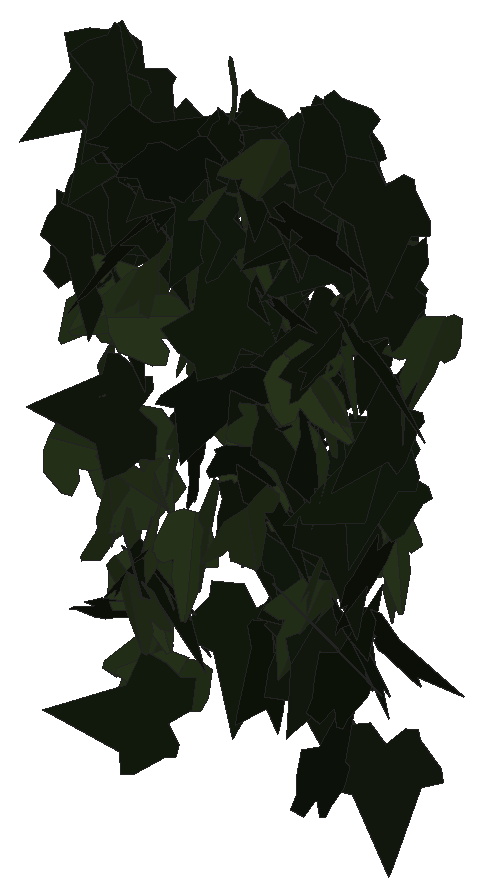
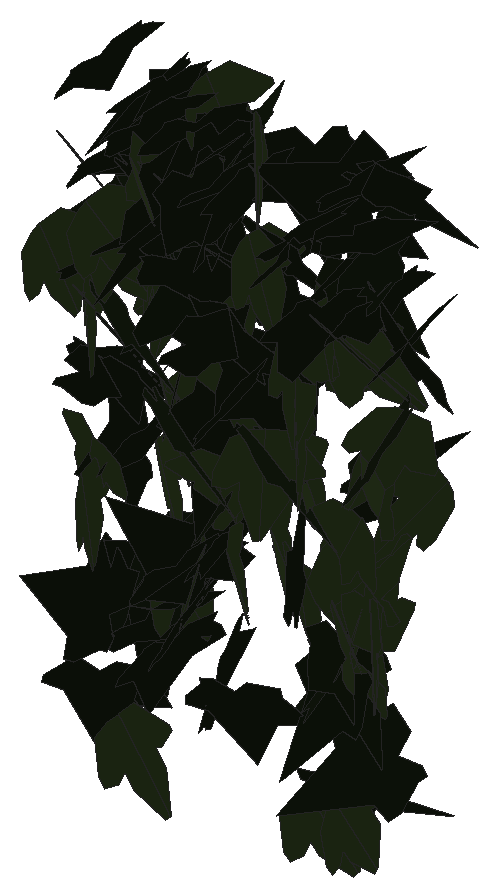
# SketchUp Ruby script. Lengths in inches.
U = 1.inch
M = Sketchup.active_model
def pt(a) = Geom::Point3d.new(a.map { |v| v * U })
def face(e, loops, mat)
  f = e.add_face(loops[0].map { |a| pt(a) })
  loops[1..].each { |l| e.add_face(l.map { |a| pt(a) }).erase! }
  f.material = f.back_material = mat if mat
  f
end
# faces: each face lists its corners as indices into pts; further lists are holes
def faces(e, pts, list, mat = nil) = list.each { |f| face(e, (f[0].is_a?(Array) ? f : [f]).map { |l| l.map { |i| pts[i] } }, mat) }
# xy, xz, yz: faces in a plane at the given z, y or x. An outline is a flat list of corners, or four numbers for a rectangle; further outlines are holes
def ring(l) = l.size == 4 ? [[l[0], l[1]], [l[2], l[1]], [l[2], l[3]], [l[0], l[3]]] : l.each_slice(2).to_a
def flat(e, list, mat, &to3) = list.each { |f| face(e, (f[0].is_a?(Array) ? f : [f]).map { |l| ring(l).map { |u, v| to3.(u, v) } }, mat) }
def xy(e, z, list, mat = nil) = flat(e, list, mat) { |x, y| [x, y, z] }
def xz(e, y, list, mat = nil) = flat(e, list, mat) { |x, z| [x, y, z] }
def yz(e, x, list, mat = nil) = flat(e, list, mat) { |y, z| [x, y, z] }
def lines(e, pts, list) = list.each { |a, b| e.add_line(pt(pts[a]), pt(pts[b])) }
# prism: a flat outline (further loops are holes) pulled along v
def prism(e, loops, v, mat = nil)
  f = face(e, loops, mat); d = Geom::Vector3d.new(v.map { |x| x * U })
  f.pushpull(f.normal.samedirection?(d) ? d.length : -d.length)
end
def box(e, o, s, mat = nil) = prism(e, [[o, [o[0] + s[0], o[1], o[2]], [o[0] + s[0], o[1] + s[1], o[2]], [o[0], o[1] + s[1], o[2]]]], [0, 0, s[2]], mat)
def at(x, y, z, deg = 0) = Geom::Transformation.translation(pt([x, y, z])) * Geom::Transformation.rotation(ORIGIN, Z_AXIS, deg.degrees)
def axes(o, x, y, z) = Geom::Transformation.new([*x, 0, *y, 0, *z, 0, *pt(o).to_a, 1])
def part(name) = M.definitions.add(name)
# library, detail: a bought-in or finely detailed component or shape, given as its bounding box
def library(name, o, s) = part(name).tap { |d| box(d.entities, o, s) }
def detail(e, o, s) = box(e.add_group.entities, o, s)
def put(e, d, t, mat = nil) = e.add_instance(d, t).tap { |i| i.material = mat if mat }
def group(e, t, mat = nil) = e.add_group.tap { |g| g.transformation = t; g.material = mat if mat }.entities
root = M.entities
M.materials.add("efeu1").color = [18, 25, 13]
M.materials.add("efeu2").color = [43, 57, 29]
c1 = part("ivyleaf_9")
p = [[1.54,2.16,1.25],[1.36,2.04,1.19],[-0.21,0.99,0.68],[-0.71,1.11,0.82],[-0.85,0.86,0.67],[-0.8,0.17,0.21],
  [-0.9,-0.01,0.1],[-0.67,-0.16,-0.02],[-0.08,-0.08,-0.05],[-0.03,-0.6,-0.4],[0.65,-0.88,-0.66],[0.83,-0.6,-0.49],
  [1.29,-0.42,-0.43],[1.8125,-0.07,-0.26],[1.21,0.44,0.15]]
faces(c1.entities,p,[[0,1,2,3,4,5,6,7,8,9,10,11,12,13,14]],"efeu1")
c2 = part("ivyleaf_10")
p = [[0,0.5,-0.03],[-0.0625,2.02,-0.43],[-0.19,2.01,-0.46],[-0.54,1.05,-0.29],[-0.52,0.625,-0.18],[-0.83,0.76,-0.28],
  [-1.16,0.64,-0.33],[-1.15,0.33,-0.24],[-0.77,-0.39,0.02],[-0.3,-0.51,0.16],[0.04,-0.48,0.23],[-0.02,2.01,-0.4375],
  [-0.06,2.01,-0.43],[0.04,-0.49,0.23],[0.67,-0.49,0.14],[1.38,0.36,-0.2],[1.375,0.51,-0.24],[0.81,0.65,-0.19],
  [0.62,0.59,-0.15],[0.6,1.09,-0.28],[0.5,1.23,-0.31]]
faces(c2.entities,p,[[0,1,2,3,4,5,6,7,8,9,10],[11,12,0,13,14,15,16,17,18,19,20]],"efeu2")
put(root,c1,axes([43.79,221.11,233.95],[-0.00332,-0.19199,0.46166],[0.22694,0.41079,0.17247],[-0.44552,0.21068,0.08441]))
put(root,c1,axes([40.89,221.49,240.28],[-0.2736,0.29374,-0.29809],[0.10434,-0.29702,-0.38845],[-0.40529,-0.27476,0.10123]))
put(root,c2,axes([42.59,221.28,237.12],[-0.08514,-0.46308,-0.16825],[0.01385,0.16843,-0.47057],[0.4925,-0.08479,-0.01586]))
put(root,c1,axes([44.14,221.52,239.85],[0.30164,-0.34888,0.19313],[0.13676,-0.13697,-0.46102],[0.37458,0.33095,0.0128]))
put(root,c2,axes([40.13,221.02,237.35],[0.08244,0.21818,0.44227],[-0.01318,0.44922,-0.21916],[-0.49298,0.02448,0.07982]))
put(root,c1,axes([40.54,221.77,237.6],[-0.02326,-0.39145,-0.31021],[0.04367,-0.31095,0.38911],[-0.49755,-0.00899,0.04865]))
put(root,c2,axes([43.27,221.34,239.25],[0.30785,0.09798,0.38161],[0.35199,0.14918,-0.32226],[-0.17701,0.46706,0.02288]))
put(root,c1,axes([43.21,221.79,237.81],[-0.00876,-0.11105,0.48743],[-0.01948,-0.48706,-0.11131],[0.49954,-0.02094,0.00421]))
put(root,c2,axes([40.78,221.57,239.25],[-0.24883,-0.09733,0.42262],[-0.34608,-0.24908,-0.26113],[0.26136,-0.42248,0.05659]))
put(root,c1,axes([43.24,221.3,241.21],[0.47749,-0.04289,0.14201],[0.14143,-0.01284,-0.47941],[0.04477,0.49799,-0.00013]))
put(root,c1,axes([43.92,221.33,239.99],[-0.31221,0.38447,0.06861],[-0.07065,0.03078,-0.49403],[-0.3841,-0.31817,0.0351]))
put(root,c2,axes([42.76,221.57,241.85],[-0.10777,-0.46898,0.13582],[-0.03653,-0.13095,-0.48116],[0.48688,-0.11364,-0.00603]))
put(root,c1,axes([43.64,221.35,239.74],[-0.36383,0.30082,0.16472],[-0.12248,0.11034,-0.47204],[-0.32035,-0.38384,-0.0066]))
put(root,c1,axes([44.3,221.7,241.87],[-0.02942,-0.498,0.03368],[-0.00026,-0.03372,-0.49886],[0.49913,-0.02937,0.00173]))
put(root,c1,axes([41.48,221.4,241.5],[0.13266,0.40843,-0.2561],[-0.06163,-0.24907,-0.42915],[-0.47812,0.14543,-0.01574]))
put(root,c1,axes([42.04,221.47,238.62],[0.07005,0.38741,-0.30823],[-0.05423,-0.30342,-0.39369],[-0.49209,0.08858,-0.00049]))
put(root,c2,axes([43.5,221.41,239.17],[-0.44305,0.23175,0.00106],[-0.00096,0.00047,-0.5],[-0.23175,-0.44305,0.00003]))
put(root,c1,axes([39.86,221.8,239.75],[0.04664,-0.47589,0.14612],[0.03164,-0.14363,-0.47788],[0.49681,0.05383,0.01672]))
put(root,c2,axes([41.12,221.46,239.87],[-0.00839,-0.48505,-0.12106],[0.01583,0.12076,-0.48494],[0.49968,-0.01197,0.01333]))
put(root,c1,axes([43.64,221.73,237.31],[0.07326,-0.49423,-0.01927],[-0.00281,0.01907,-0.49963],[0.4946,0.07331,0.00001]))
put(root,c2,axes([40.79,221.35,239.07],[-0.0798,-0.05196,0.49085],[0.3641,0.32952,0.09407],[-0.33326,0.37245,-0.01475]))
put(root,c1,axes([42.3,221.49,239.24],[-0.46284,-0.17411,0.07395],[0.07953,-0.00177,0.49363],[-0.17163,0.4687,0.02933]))
put(root,c2,axes([40.29,221.76,235.96],[-0.03633,-0.45845,-0.19623],[-0.02154,-0.19512,0.45985],[-0.49821,0.04187,-0.00558]))
put(root,c1,axes([42.14,221.88,241.54],[0.07074,-0.40837,0.27969],[0.10376,-0.26402,-0.41174],[0.48397,0.1163,0.04739]))
put(root,c2,axes([43.48,221.58,236.875],[0.21909,-0.44116,-0.08587],[-0.04545,0.0733,-0.49251],[0.44714,0.22361,-0.00798]))
put(root,c1,axes([44.22,221.16,236.63],[0.05923,0.16627,0.46781],[0.1305,0.44935,-0.17623],[-0.47902,0.14297,0.00983]))
put(root,c2,axes([43.61,221.76,239.66],[-0.23912,0.20358,-0.38907],[0.22364,-0.3248,-0.30739],[-0.3779,-0.32103,0.06428]))
put(root,c1,axes([42.82,221.81,238.04],[0.1355,-0.47363,0.08555],[0.03131,-0.08001,-0.49256],[0.48027,0.13884,0.00797]))
put(root,c1,axes([40.98,221.75,233.63],[-0.3539,0.13637,0.32581],[-0.34847,-0.05961,-0.35357],[-0.05759,-0.47734,0.13723]))
put(root,c2,axes([41.36,221.75,236.26],[0.46537,-0.12615,0.13235],[0.1254,-0.04316,-0.48209],[0.13305,0.4819,-0.00854]))
put(root,c1,axes([43.8125,221.41,235.04],[-0.02848,-0.15028,0.47603],[0.23675,0.4157,0.1454],[-0.43947,0.23369,0.04747]))
put(root,c2,axes([42.61,221.68,238.21],[-0.4778,-0.07243,-0.12828],[0.13851,-0.07254,-0.47493],[0.05019,-0.48938,0.08938]))
put(root,c2,axes([40.67,221.59,235.39],[-0.47041,0.14948,0.07982],[-0.07614,0.02394,-0.49359],[-0.15138,-0.47653,0.00024]))
put(root,c1,axes([40.67,221.73,240.54],[0.19733,-0.43666,-0.14278],[-0.02891,0.14329,-0.47816],[0.4585,0.19697,0.0313]))
put(root,c2,axes([41.57,221.91,236.67],[0.22492,-0.33764,0.29224],[0.21177,-0.20743,-0.40265],[0.39314,0.30491,0.0497]))
put(root,c2,axes([43.36,221.65,237.81],[0.29069,-0.34861,-0.20969],[-0.13111,0.16369,-0.45389],[0.38511,0.31887,0.00375]))
put(root,c1,axes([40.66,221.49,241.07],[0.09315,-0.01824,0.49091],[0.47311,0.13785,-0.08465],[-0.13226,0.48027,0.04294]))
put(root,c1,axes([39.83,221.58,239.28],[-0.31379,0.30985,0.23564],[0.15863,-0.17462,0.44084],[0.35549,0.35143,0.01129]))
put(root,c2,axes([40.65,221.57,235.96],[-0.28288,0.38532,0.14666],[-0.10541,0.10435,-0.47749],[-0.39858,-0.30107,0.0222]))
put(root,c1,axes([44.28,222.02,237.95],[-0.39156,-0.16392,0.26421],[-0.24333,-0.10296,-0.42449],[0.19357,-0.46101,0.00086]))
put(root,c2,axes([41.2,221.9,237.74],[0.23088,-0.42641,0.12195],[0.06976,-0.10085,-0.48473],[0.43798,0.24085,0.01292]))
put(root,c2,axes([40.61,221.99,236.34],[-0.2559,-0.18987,-0.38531],[-0.3177,-0.2182,0.31852],[-0.2891,0.40785,-0.00897]))
put(root,c1,axes([42.6,222.17,241.18],[-0.16978,-0.3912,0.26103],[-0.00302,-0.27661,-0.41651],[0.47028,-0.14301,0.09156]))
put(root,c1,axes([42.25,222.16,234.78],[0.12546,-0.19063,-0.44488],[0.35566,-0.2754,0.21831],[-0.32827,-0.37123,0.06649]))
put(root,c1,axes([39.99,221.83,240.91],[0.4044,-0.27652,0.09999],[0.0764,-0.06538,-0.48978],[0.28394,0.41142,-0.01062]))
put(root,c1,axes([40.18,221.98,241.84],[-0.48772,-0.0446,0.1007],[-0.09851,-0.02774,-0.48941],[0.04924,-0.49723,0.01828]))
put(root,c1,axes([42.89,221.79,235.84],[0.42394,-0.2403,0.11196],[0.11473,-0.02407,-0.48606],[0.23899,0.43781,0.03473]))
put(root,c1,axes([44.59,221.83,240.6],[-0.45342,0.20912,0.02606],[-0.02396,0.01026,-0.49932],[-0.20938,-0.45405,0.00071]))
put(root,c1,axes([40.3,222.18,241.84],[-0.21736,-0.40657,0.19354],[-0.01371,-0.20884,-0.45409],[0.45008,-0.20271,0.07964]))
put(root,c1,axes([44.39,221.9375,238.86],[-0.47957,0.11835,-0.07752],[0.06961,-0.04112,-0.49342],[-0.12317,-0.48405,0.02296]))
put(root,c1,axes([43.97,222.04,238.2],[-0.39118,-0.17873,-0.25502],[0.26599,0.02116,-0.42285],[0.16195,-0.46648,0.07853]))
put(root,c1,axes([41.33,222.22,240.51],[-0.08097,-0.41561,0.26591],[-0.03918,-0.2632,-0.42331],[0.49184,-0.08939,0.01006]))
put(root,c1,axes([42.43,221.6,237.84],[0.27374,0.41687,-0.03582],[-0.01431,-0.03345,-0.49867],[-0.41816,0.27404,-0.00639]))
put(root,c2,axes([42.94,222.08,235.81],[-0.04783,-0.43246,0.24635],[0.03738,-0.24991,-0.43145],[0.4963,-0.02285,0.05624]))
put(root,c1,axes([42.68,222,241.68],[-0.10361,-0.45867,-0.16995],[0.04713,0.16355,-0.47014],[0.48687,-0.11344,0.00934]))
put(root,c1,axes([40.05,222.11,240.38],[-0.00182,-0.49977,-0.01512],[0.0009,0.01512,-0.49977],[0.5,-0.00185,0.00085]))
put(root,c1,axes([42.7,221.78,239.66],[0.49509,-0.06971,-0.00542],[-0.00469,0.00555,-0.49995],[0.06976,0.49509,0.00484]))
put(root,c1,axes([43.51,222.17,235.43],[0.16893,-0.3269,0.33853],[0.15985,-0.29843,-0.36795],[0.44262,0.23254,0.00368]))
put(root,c1,axes([41.77,221.97,240.48],[-0.45258,0.12552,0.1715],[-0.16748,0.03773,-0.4696],[-0.13083,-0.48251,0.00789]))
put(root,c1,axes([42.16,222.06,237.22],[0.28945,-0.40566,0.04073],[0.02525,-0.03201,-0.49833],[0.40692,0.29054,0.00195]))
put(root,c1,axes([44.01,222.07,234.19],[-0.26835,-0.32907,-0.26401],[0.17959,0.19402,-0.42439],[0.38175,-0.32259,0.01406]))
put(root,c2,axes([40.5625,221.86,235.46],[0.33819,-0.34502,0.12879],[-0.07308,0.1085,0.48258],[-0.36095,-0.34524,0.02296]))
put(root,c2,axes([40.46,221.97,235.39],[0.41922,0.00792,0.27238],[0.2696,0.06058,-0.41671],[-0.0396,0.49625,0.04653]))
put(root,c1,axes([40.15,222.3,241.29],[-0.33528,-0.36132,0.08388],[0.00337,-0.11603,-0.48634],[0.37091,-0.32555,0.08024]))
put(root,c2,axes([40.47,222.03,237.23],[-0.43642,0.08709,-0.22792],[0.19344,-0.16116,-0.43198],[-0.14871,-0.46523,0.10697]))
put(root,c1,axes([43.5,222.1,240.85],[-0.49442,0.0652,0.03609],[-0.03854,-0.01643,-0.49824],[-0.06378,-0.49546,0.02127]))
put(root,c1,axes([41.05,222.39,240.96],[-0.25673,-0.33094,0.27307],[-0.05418,-0.29068,-0.4032],[0.42562,-0.23662,0.11339]))
put(root,c2,axes([42,222.09,240.08],[-0.32782,0.11036,-0.36104],[0.30149,-0.21126,-0.33833],[-0.22723,-0.43953,0.07197]))
put(root,c1,axes([43.11,222.33,235.31],[-0.21591,-0.43449,0.12085],[-0.01504,-0.12697,-0.48338],[0.45073,-0.21236,0.04176]))
put(root,c1,axes([40.57,222.08,235.53],[0.30692,-0.39364,-0.02915],[-0.02235,0.01953,-0.49912],[0.39408,0.30769,-0.00561]))
put(root,c2,axes([39.79,222.375,238],[-0.06161,-0.1328,-0.47809],[0.11549,-0.47237,0.11632],[-0.48256,-0.09609,0.08888]))
put(root,c1,axes([42.04,222.16,236.75],[0.13615,-0.47305,-0.0877],[-0.03475,0.08124,-0.49213],[0.47985,0.1401,-0.01076]))
put(root,c2,axes([42.95,222.05,241.11],[-0.37177,-0.33335,0.02588],[-0.0104,-0.02715,-0.49915],[0.33419,-0.37168,0.01326]))
put(root,c1,axes([40.62,221.95,235.7],[-0.17864,0.45943,-0.08372],[0.02797,-0.07895,-0.49293],[-0.46616,-0.1808,0.00251]))
put(root,c2,axes([44.34,221.88,238.96],[0.28801,-0.23563,-0.33396],[-0.14247,0.32504,-0.35221],[0.38308,0.29804,0.12009]))
put(root,c2,axes([44.02,222.16,237.13],[0.43026,-0.10607,0.23158],[0.22996,-0.03375,-0.4427],[0.10954,0.48745,0.01974]))
put(root,c1,axes([42.98,222.47,240.88],[-0.08397,-0.12251,-0.47743],[0.17302,-0.46082,0.08782],[-0.46153,-0.15046,0.11979]))
put(root,c2,axes([43.65,222.35,239.99],[0.0134,-0.4241,0.2645],[0.01752,-0.26403,-0.42424],[0.49951,0.02064,0.00779]))
put(root,c1,axes([42.89,222.22,235.02],[0.02485,-0.47679,-0.14849],[-0.02184,0.1475,-0.47725],[0.4989,0.03021,-0.0135]))
put(root,c1,axes([43.1,222.46,241.75],[-0.21632,-0.43098,0.13215],[-0.03066,-0.13218,-0.48124],[0.44974,-0.21631,0.03076]))
put(root,c1,axes([42.43,221.95,241.55],[0.31678,0.25463,-0.29122],[-0.27566,-0.1155,-0.40084],[-0.2714,0.41452,0.06721]))
put(root,c1,axes([43.17,222.27,242.04],[0.13714,-0.4784,-0.0482],[-0.01042,0.04716,-0.49766],[0.48071,0.1375,0.00296]))
put(root,c1,axes([42.3,222.38,239.48],[0.13259,-0.46298,0.13444],[0.02464,-0.13274,-0.48143],[0.48147,0.13429,-0.01238]))
put(root,c2,axes([39.82,222.03,238.75],[-0.23047,-0.35749,-0.26285],[0.20539,0.17659,-0.42027],[0.39332,-0.30169,0.06545]))
put(root,c1,axes([43.57,222.47,241.28],[-0.06292,-0.48359,0.11037],[0.00967,-0.11243,-0.4871],[0.49593,-0.05916,0.0235]))
put(root,c2,axes([42.32,222.32,241.08],[-0.13962,-0.45414,0.15578],[-0.02151,-0.15615,-0.4745],[0.47963,-0.1392,0.02407]))
put(root,c1,axes([43.07,222.11,242.125],[0.19767,-0.373,-0.26795],[0.0167,0.29736,-0.40162],[0.45897,0.14983,0.13001]))
put(root,c1,axes([42.24,222.1,239.18],[-0.26118,0.17998,0.38651],[-0.33594,0.19225,-0.31652],[-0.26255,-0.42502,0.0205]))
put(root,c1,axes([40.5,222.04,235.36],[0.48037,-0.02626,-0.13622],[-0.13605,0.0069,-0.48109],[0.02714,0.49926,-0.00051]))
put(root,c1,axes([40.56,222.35,239.97],[-0.48779,0.09455,-0.05584],[0.03897,-0.08861,-0.49054],[-0.10266,-0.48292,0.07908]))
put(root,c1,axes([42.14,222.43,241.24],[-0.03856,-0.49848,-0.00593],[-0.00045,0.00598,-0.49996],[0.49851,-0.03855,-0.00091]))
put(root,c2,axes([42.11,222.21,237.51],[0.43566,0.21406,0.11992],[0.11366,0.04051,-0.48522],[-0.21745,0.45004,-0.01336]))
put(root,c2,axes([44.48,222.41,239.71],[-0.06923,-0.46222,0.17764],[0.02118,-0.18197,-0.46523],[0.49473,-0.05689,0.04478]))
put(root,c1,axes([39.69,222.45,238.71],[0.20657,-0.4283,0.15455],[0.06188,-0.14173,-0.47548],[0.45111,0.21557,-0.00554]))
put(root,c1,axes([41.84,222.62,238.59],[-0.06935,-0.39317,0.30101],[-0.01696,-0.30188,-0.39822],[0.49488,-0.06544,0.02853]))
put(root,c1,axes([42.57,222.49,236.26],[-0.10913,-0.48791,0.00628],[-0.00486,-0.00535,-0.49995],[0.48792,-0.10918,-0.00358]))
put(root,c1,axes([43.75,222.3,239.23],[-0.42914,0.23722,-0.09778],[0.07638,-0.06381,-0.48999],[-0.24496,-0.43549,0.01853]))
put(root,c2,axes([40.18,222.49,233.9],[-0.02494,-0.4247,0.26269],[0.07713,-0.26313,-0.4181],[0.49338,0.01967,0.07864]))
put(root,c2,axes([40.625,222.45,233.83],[-0.23441,-0.36341,0.25097],[-0.0592,-0.25571,-0.42557],[0.43766,-0.22923,0.07686]))
put(root,c1,axes([42.3125,222.6,239.26],[-0.30692,-0.23689,0.31572],[-0.2475,-0.19605,-0.3877],[0.30748,-0.39427,0.00309]))
put(root,c2,axes([41.08,222.21,239.35],[-0.03558,-0.4805,-0.13361],[0.00084,0.13389,-0.48174],[0.49873,-0.0345,-0.00872]))
put(root,c2,axes([41.52,222.4,240.57],[-0.01483,-0.49607,0.06076],[0.00333,-0.06088,-0.49627],[0.49977,-0.01432,0.00511]))
put(root,c2,axes([40.01,222.15,236.28],[0.23825,-0.33309,-0.28687],[-0.08707,0.28407,-0.40215],[0.43088,0.24158,0.07735]))
put(root,c2,axes([43.08,222.54,241.23],[0.26531,-0.294,0.30525],[0.20779,-0.22364,-0.39599],[0.36937,0.33697,0.00351]))
put(root,c1,axes([43.6,222.7,239.98],[-0.24941,-0.38955,0.18985],[-0.00303,-0.21748,-0.45022],[0.43334,-0.22572,0.10612]))
put(root,c1,axes([41.51,222.31,238.1],[-0.38889,0.31406,0.01137],[-0.02729,-0.01573,-0.49901],[-0.31308,-0.38874,0.02937]))
put(root,c2,axes([41.48,222.32,238.03],[-0.35751,-0.349,-0.01969],[0.01844,0.0093,-0.49957],[0.34907,-0.35793,0.00622]))
put(root,c2,axes([41.65,222.19,241.98],[0.21844,-0.34055,-0.29379],[-0.0869,0.2885,-0.39902],[0.44128,0.22539,0.06685]))
put(root,c1,axes([42.48,222.75,235.47],[-0.13615,-0.19287,0.44075],[-0.07362,-0.44432,-0.21717],[0.47544,-0.12403,0.09259]))
put(root,c1,axes([42.46,222.2,236.07],[-0.09732,-0.02968,0.48954],[0.488,0.04384,0.09967],[-0.04884,0.49719,0.02043]))
put(root,c2,axes([42.41,222.36,236.34],[-0.27904,0.40509,-0.08965],[0.04109,-0.08052,-0.49176],[-0.41285,-0.28181,0.01165]))
put(root,c1,axes([42.43,222.62,240.28],[-0.36662,-0.33558,-0.05459],[0.04022,0.0369,-0.49701],[0.3376,-0.36882,-0.00006]))
put(root,c2,axes([43.87,222.49,236.74],[0.14882,-0.46961,0.08553],[0.11675,-0.05106,-0.48349],[0.46284,0.16388,0.09446]))
put(root,c1,axes([41.67,222.56,234.96],[-0.34384,-0.29795,-0.20736],[0.16843,0.12206,-0.45468],[0.32157,-0.38252,0.01643]))
put(root,c1,axes([39.81,222.08,234.6],[0.45187,0.12208,0.17582],[0.11667,0.20384,-0.4414],[-0.17945,0.43994,0.15573]))
put(root,c1,axes([42.31,222.5,241.29],[-0.1386,0.33963,-0.33977],[0.11131,-0.3213,-0.36657],[-0.46733,-0.17725,0.01346]))
put(root,c1,axes([41.63,222.33,241.53],[0.16564,-0.36514,-0.29873],[-0.10263,0.28113,-0.40054],[0.46047,0.19401,0.01819]))
put(root,c1,axes([43.59,222.51,235.32],[0.26706,-0.21699,0.36276],[0.30367,-0.20001,-0.34319],[0.29405,0.40362,0.02496]))
put(root,c1,axes([42.86,222.41,238.15],[-0.41346,0.27978,-0.02781],[0.02389,-0.01431,-0.49922],[-0.28014,-0.41415,-0.00153]))
put(root,c2,axes([40.92,222.38,238.67],[0.22524,-0.43116,-0.11562],[0.02253,0.14032,-0.47938],[0.44582,0.21074,0.08264]))
put(root,c1,axes([40.57,222.42,240.22],[0.02018,-0.41124,-0.28368],[-0.01803,0.28313,-0.41172],[0.49927,0.02685,-0.0034]))
put(root,c2,axes([43.57,222.64,240.43],[-0.13837,-0.39695,0.27071],[-0.06779,-0.26277,-0.41995],[0.47567,-0.15292,0.0189]))
put(root,c2,axes([43.35,222.44,233.78],[-0.34497,-0.05243,0.35812],[-0.35469,-0.04954,-0.34891],[0.07207,-0.49477,-0.00301]))
put(root,c2,axes([41.61,222.66,236.69],[0.2787,-0.32967,0.25229],[0.18855,-0.17019,-0.43068],[0.36984,0.33519,0.02945]))
put(root,c1,axes([40.73,222.71,236.55],[-0.01932,0.15749,0.47416],[-0.05132,-0.47263,0.15489],[0.49698,-0.04268,0.03443]))
put(root,c1,axes([42.8,222.37,240.59],[0.22439,-0.32983,-0.30143],[-0.07333,0.30555,-0.38892],[0.44076,0.21875,0.08875]))
